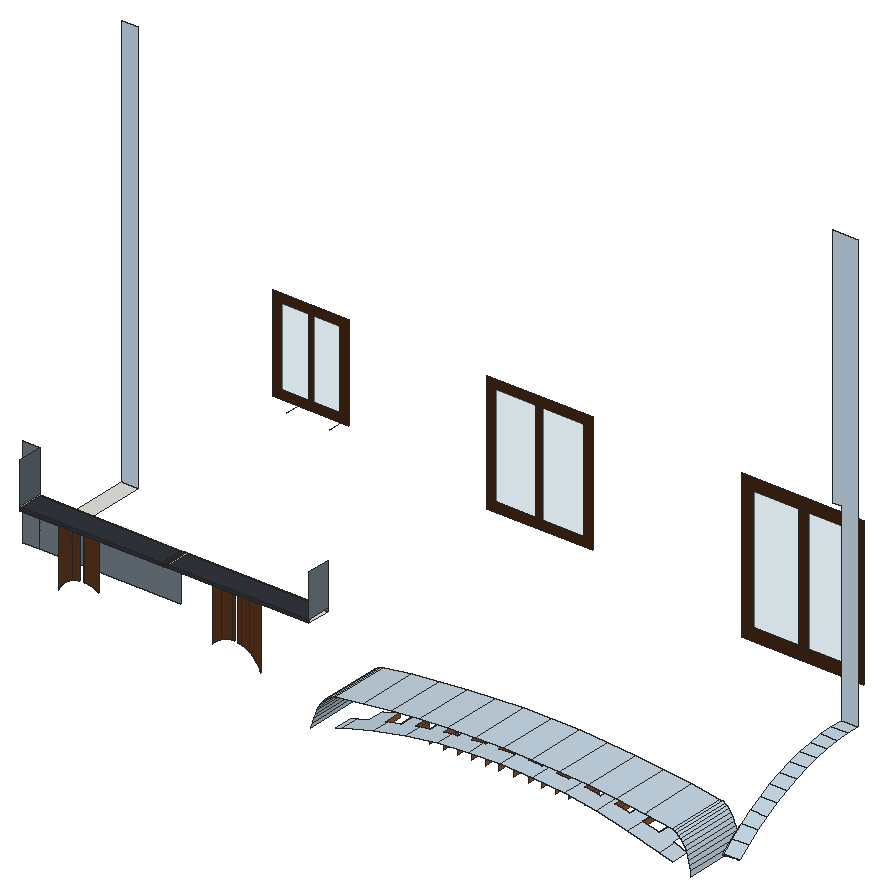
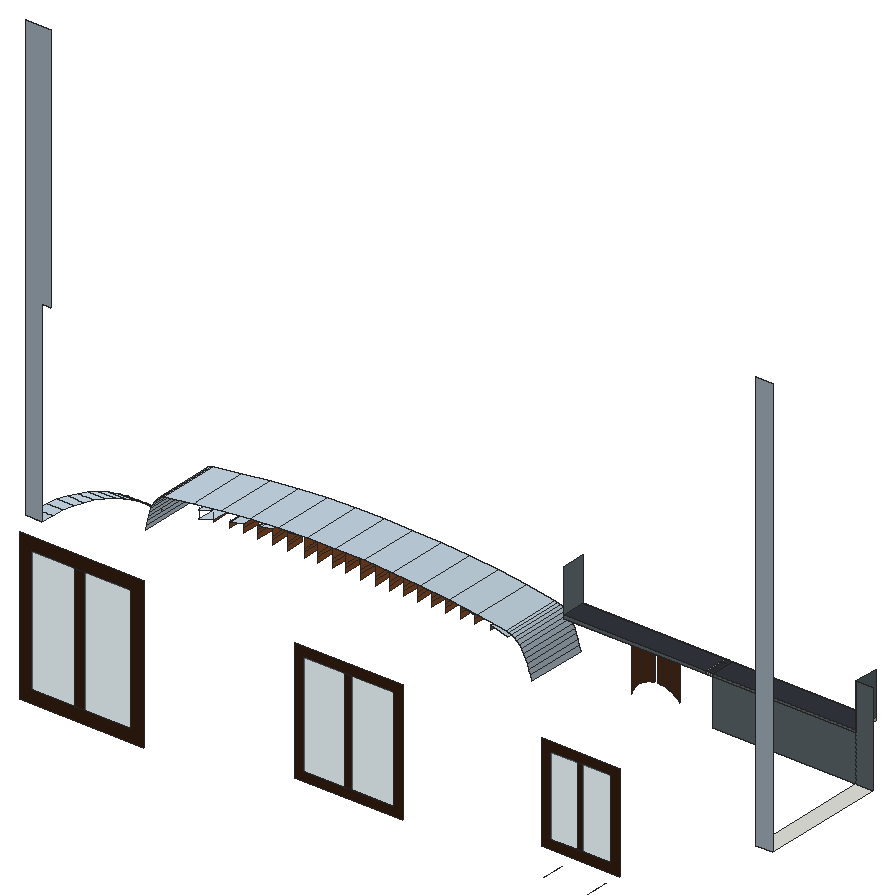
# SketchUp Ruby script. Lengths in inches.
U = 1.inch
M = Sketchup.active_model
def pt(a) = Geom::Point3d.new(a.map { |v| v * U })
def face(e, loops, mat)
  f = e.add_face(loops[0].map { |a| pt(a) })
  loops[1..].each { |l| e.add_face(l.map { |a| pt(a) }).erase! }
  f.material = f.back_material = mat if mat
  f
end
# faces: each face lists its corners as indices into pts; further lists are holes
def faces(e, pts, list, mat = nil) = list.each { |f| face(e, (f[0].is_a?(Array) ? f : [f]).map { |l| l.map { |i| pts[i] } }, mat) }
# xy, xz, yz: faces in a plane at the given z, y or x. An outline is a flat list of corners, or four numbers for a rectangle; further outlines are holes
def ring(l) = l.size == 4 ? [[l[0], l[1]], [l[2], l[1]], [l[2], l[3]], [l[0], l[3]]] : l.each_slice(2).to_a
def flat(e, list, mat, &to3) = list.each { |f| face(e, (f[0].is_a?(Array) ? f : [f]).map { |l| ring(l).map { |u, v| to3.(u, v) } }, mat) }
def xy(e, z, list, mat = nil) = flat(e, list, mat) { |x, y| [x, y, z] }
def xz(e, y, list, mat = nil) = flat(e, list, mat) { |x, z| [x, y, z] }
def yz(e, x, list, mat = nil) = flat(e, list, mat) { |y, z| [x, y, z] }
def lines(e, pts, list) = list.each { |a, b| e.add_line(pt(pts[a]), pt(pts[b])) }
# prism: a flat outline (further loops are holes) pulled along v
def prism(e, loops, v, mat = nil)
  f = face(e, loops, mat); d = Geom::Vector3d.new(v.map { |x| x * U })
  f.pushpull(f.normal.samedirection?(d) ? d.length : -d.length)
end
def box(e, o, s, mat = nil) = prism(e, [[o, [o[0] + s[0], o[1], o[2]], [o[0] + s[0], o[1] + s[1], o[2]], [o[0], o[1] + s[1], o[2]]]], [0, 0, s[2]], mat)
def at(x, y, z, deg = 0) = Geom::Transformation.translation(pt([x, y, z])) * Geom::Transformation.rotation(ORIGIN, Z_AXIS, deg.degrees)
def axes(o, x, y, z) = Geom::Transformation.new([*x, 0, *y, 0, *z, 0, *pt(o).to_a, 1])
def part(name) = M.definitions.add(name)
# library, detail: a bought-in or finely detailed component or shape, given as its bounding box
def library(name, o, s) = part(name).tap { |d| box(d.entities, o, s) }
def detail(e, o, s) = box(e.add_group.entities, o, s)
def put(e, d, t, mat = nil) = e.add_instance(d, t).tap { |i| i.material = mat if mat }
def group(e, t, mat = nil) = e.add_group.tap { |g| g.transformation = t; g.material = mat if mat }.entities
root = M.entities
M.materials.add("[Formica Laminate Dark]").color = [50, 53, 60]
M.materials.add("[Formica Speckled Grey]").color = [110, 123, 130]
M.materials.add("[Formica Speckled Grey]1").color = [94, 105, 111]
M.materials.add("[Terrazzo Light Blue]").color = [196, 214, 227]
M.materials.add("[Translucent Glass Safety]").color = [204, 235, 244]
M.materials["[Translucent Glass Safety]"].alpha = 0.5
M.materials.add("[Wood Cherry Original]").color = [152, 86, 42]
M.materials.add("[Wood Veneer 01]1").color = [86, 50, 26]
M.materials.add("[Wood Veneer 01]2").color = [63, 37, 19]
xy(root,128.61,[[0,134.14,19.68,283.27]])
xy(root,183.04,[[19.68,105.19,190.08,134.14],[190.08,105.19,198.05,134.14],[198.05,105.19,367.43,134.14]])
xy(root,186.5625,[[19.68,105.19,190.08,134.14],[190.08,105.19,193.18,134.14],[193.18,105.19,194.95,134.14],[194.95,105.19,198.05,134.14],[198.05,105.19,367.43,134.14]],"[Formica Laminate Dark]")
xz(root,105.19,[[868.09,108.42,887.77,109.72,868.09,109.72]])
xz(root,105.19,[[19.68,183.04,190.08,186.5625],[190.08,183.04,193.18,186.5625],[193.18,183.04,194.95,186.5625],[194.95,183.04,198.05,186.5625],[198.05,183.04,367.43,186.5625]],"[Formica Laminate Dark]")
xz(root,105.19,[[310.25,109.72,310.25,183.04,296.83,183.04,296.83,127.07,298.1,126.25,300.86,124.02,303.36,121.51,305.59,118.76,307.53,115.78,309.13,112.625],[65.75,113.31,65.96,113.76,66.33,114.49,66.71,115.2,67.11,115.91,67.53,116.61,67.97,117.3,68.42,117.97,68.88,118.64,69.37,119.29,69.87,119.93,70.38,120.5625,70.91,121.18,71.45,121.79,72.01,122.38,72.58,122.96,73.17,123.52,73.76,124.07,74.375,124.6,75,125.125,75.64,125.63,76.29,126.12,76.95,126.59,77.62,127.05,78.3,127.49,78.99,127.92,79.7,128.33,80.41,128.72,81.13,129.1,81.86,129.45,81.93,129.49,81.93,183.04,65.75,183.04],[252.33,120.67,253.01,121.51,255.52,124.02,258.28,126.25,261.25,128.18,263.46,129.31,263.46,183.04,252.33,183.04],[296.83,127.07,296.83,183.04,285.71,183.04,285.71,131.85,288.66,131.0625,291.97,129.79,295.125,128.18],[114.31,127.58,114.31,183.04,98.12,183.04,98.12,132.68,98.15,132.67,99.03,132.62,99.92,132.53,100.8,132.43,101.68,132.3,102.55,132.15,103.42,131.98,104.28,131.78,105.14,131.57,106,131.33,106.84,131.0625,107.68,130.78,108.52,130.47,109.34,130.14,110.15,129.79,110.96,129.42,111.75,129.03,112.54,128.62,113.3125,128.18,114.08,127.73],
  [263.46,129.31,264.41,129.79,267.72,131.0625,271.15,131.98,274.58,132.52,274.58,183.04,263.46,183.04],[81.93,129.49,82.6,129.79,83.34,130.11,84.1,130.42,84.86,130.7,85.63,130.97,86.4,131.22,87.18,131.45,87.97,131.66,88.76,131.85,89.55,132.03,90.35,132.18,91.15,132.31,91.99,132.14,91.99,183.04,81.93,183.04],[285.71,131.85,285.71,183.04,282.74,183.04,282.74,132.375,285.23,131.98],[274.58,132.52,274.65,132.53,278.1875,132.72,278.36,132.71,278.36,183.04,274.58,183.04],[98.12,132.68,98.12,183.04,96.375,183.04,96.375,132.72,97.26,132.71]],"[Wood Veneer 01]1")
xz(root,134.14,[[190.08,183.04,193.18,186.5625],[193.18,183.04,194.95,186.5625],[194.95,183.04,198.05,186.5625]])
xz(root,134.14,[[0,128.61,19.68,238.16],[19.68,128.61,190.08,183.04],[19.68,183.04,190.08,186.5625],[198.05,183.04,367.43,186.5625]],"[Formica Speckled Grey]")
xz(root,283.27,[[0,128.61,19.68,627.66],[868.09,175.78,887.77,175.78,887.77,702.66,857.52,702.66,857.52,407.22,868.09,407.22]],"[Terrazzo Light Blue]")
xz(root,454.3,[[625.86,115.33,680.16,263.36],[692.53,115.33,743.14,263.36],[313.91,142.1875,362.85,264.26],[371.15,142.1875,420.11,264.26],[55.54,172.47,88.73,266.53],
  [94.98,172.47,126.6,266.53]],"[Translucent Glass Safety]")
xz(root,454.3,[[[611.1,100.57,757.91,278.13],[625.86,115.33,743.14,263.36]],[680.16,115.33,692.53,263.36],[[303.04,131.32,430.98,275.13],[313.91,142.1875,420.11,264.26]],[362.85,142.1875,371.15,264.26],[[45.16,162.09,136.97,276.9],[55.54,172.47,126.6,266.53]],
  [88.73,172.47,94.98,266.53]],"[Wood Veneer 01]2")
yz(root,19.68,[[105.19,183.04,134.14,186.5625]])
yz(root,19.68,[[105.19,186.5625,134.14,238.16]],"[Formica Speckled Grey]1")
yz(root,190.08,[[105.19,183.04,134.14,186.5625]])
yz(root,198.05,[[105.19,183.04,134.14,186.5625]])
yz(root,367.43,[[105.19,186.5625,134.14,238.16]],"[Formica Speckled Grey]")
yz(root,477.51,[[84.44,119.05,105.19,124.6]],"[Wood Cherry Original]")
yz(root,495.83,[[84.44,119.05,105.19,124.6],[84.44,124.6,105.19,128.67]],"[Wood Cherry Original]")
yz(root,513.14,[[84.44,132.11,105.19,132.3]])
yz(root,513.14,[[84.44,119.05,105.19,124.6],[84.44,124.6,105.19,128.67],[84.44,128.67,105.19,132.11]],"[Wood Cherry Original]")
yz(root,530.58,[[84.44,119.05,105.19,124.6],[84.44,124.6,105.19,128.67],[84.44,128.67,105.19,135.3]],"[Wood Cherry Original]")
yz(root,547.58,[[84.44,119.05,105.19,124.6],[84.44,124.6,105.19,128.67],[84.44,128.67,105.19,137.84]],"[Wood Cherry Original]")
yz(root,564.14,[[84.44,119.05,105.19,124.6],[84.44,124.6,105.19,128.67],[84.44,128.67,105.19,139.94]],"[Wood Cherry Original]")
yz(root,580.83,[[84.44,119.05,105.19,124.6],[84.44,124.6,105.19,128.67],[84.44,128.67,105.19,141.4375]],"[Wood Cherry Original]")
yz(root,597.64,[[84.44,119.05,105.19,124.6],[84.44,124.6,105.19,128.67],[84.44,128.67,105.19,142.86]],"[Wood Cherry Original]")
yz(root,613.45,[[84.44,119.05,105.19,124.6],[84.44,124.6,105.19,128.67],[84.44,128.67,105.19,143.33]],"[Wood Cherry Original]")
yz(root,631.83,[[84.44,119.05,105.19,124.6],[84.44,124.6,105.19,128.67],[84.44,128.67,105.19,143.88]],"[Wood Cherry Original]")
yz(root,650.26,[[84.44,119.05,105.19,124.6],[84.44,124.6,105.19,128.67],[84.44,128.67,105.19,143.5]],"[Wood Cherry Original]")
yz(root,665.7,[[84.44,119.05,105.19,124.6],[84.44,124.6,105.19,128.67],[84.44,128.67,105.19,143.04]],"[Wood Cherry Original]")
yz(root,683.14,[[84.44,119.05,105.19,124.6],[84.44,124.6,105.19,128.67],[84.44,128.67,105.19,141.91]],"[Wood Cherry Original]")
yz(root,698.33,[[84.44,119.05,105.19,124.6],[84.44,124.6,105.19,128.67],[84.44,128.67,105.19,140.55]],"[Wood Cherry Original]")
yz(root,718.2,[[84.44,119.05,105.19,124.6],[84.44,124.6,105.19,128.67],[84.44,128.67,105.19,138.35]],"[Wood Cherry Original]")
yz(root,736.39,[[84.44,119.05,105.19,124.6],[84.44,124.6,105.19,128.67],[84.44,128.67,105.19,135.63]],"[Wood Cherry Original]")
yz(root,754.39,[[84.44,119.05,105.19,124.6],[84.44,124.6,105.19,128.67],[84.44,128.67,105.19,132.65]],"[Wood Cherry Original]")
yz(root,771.39,[[84.44,119.05,105.19,124.6],[84.44,124.6,105.19,128.67],[84.44,128.67,105.19,129.09]],"[Wood Cherry Original]")
yz(root,787.33,[[84.44,119.05,105.19,124.6],[84.44,124.6,105.19,125.74]],"[Wood Cherry Original]")
yz(root,806.7,[[84.44,119.05,105.19,120.53]],"[Wood Cherry Original]")
yz(root,868.09,[[105.19,108.42,105.19,109.72,118.73,120.31,130.3,128.41,118.54,119.63,107.97,110.74]])
p = [[405.48,134.14,102.81],[405.48,61.94,102.81],[406.89,61.94,108.68],[406.89,134.14,108.68],[863.19,134.14,108.38],[863.19,61.94,108.38],
  [863.71,61.94,102.81],[863.71,134.14,102.81],[862.36,134.14,113.8],[862.36,61.94,113.8],[408.5625,61.94,114.26],[408.5625,134.14,114.26],
  [887.77,105.19,109.72],[887.77,118.73,120.31],[868.09,118.73,120.31],[868.09,105.19,109.72],[825.83,61.94,115.36],[825.83,84.44,115.36],
  [841.21,84.44,110.27],[841.21,61.94,110.27],[435.4375,61.94,112.74],[435.4375,84.44,112.74],[443.36,84.44,115.36],[443.36,61.94,115.36],
  [861.24,134.14,118.99],[861.24,61.94,118.99],[410.48,61.94,119.51],[410.48,134.14,119.51],[457.01,84.44,119.05],[457.01,105.19,119.05],
  [477.51,105.19,124.6],[477.51,84.44,124.6],[481.41,84.44,125.65],[481.41,61.94,125.65],[787.78,61.94,125.65],[787.78,84.44,125.65],
  [806.7,84.44,120.53],[806.7,105.19,120.53],[823.96,105.19,115.87],[823.96,84.44,115.87],[859.83,134.14,123.88],[859.83,61.94,123.88],
  [412.62,61.94,124.4],[412.62,134.14,124.4],[887.77,132.61,130.03],[868.09,132.61,130.03],[868.09,130.3,128.41],[858.16,134.14,128.43],
  [858.16,61.94,128.43],[414.96,61.94,128.87],[414.96,134.14,128.87],[495.83,84.44,128.67],[495.83,105.19,128.67],[513.14,105.19,132.3],
  [513.14,84.44,132.3],[519.59,84.44,133.66],[519.59,61.94,133.66],[749.6,105.19,133.66],[754.39,105.19,132.65],[754.39,84.44,132.65],
  [771.39,84.44,129.09],[771.39,105.19,129.09],[787.33,105.19,125.74],[787.33,84.44,125.74],[749.6,61.94,133.66],[856.24,134.14,132.55],
  [856.24,61.94,132.55],[417.5,61.94,132.89],[417.5,134.14,132.89],[887.77,146.79,138.86],[868.09,146.79,138.86],[854.11,134.14,136.22],
  [854.11,61.94,136.22],[420.2,61.94,136.44],[420.2,134.14,136.44],[530.58,84.44,135.3],[530.58,105.19,135.3],[547.58,105.19,137.84],
  [547.58,84.44,137.84],[557.87,84.44,139.38],[557.87,61.94,139.38],[711.32,105.19,139.38],[718.2,105.19,138.35],[718.2,84.44,138.35],
  [736.39,84.44,135.63],[736.39,105.19,135.63],[711.32,61.94,139.38],[851.78,134.14,139.36],[851.78,61.94,139.36],[423.05,61.94,139.48],
  [423.05,134.14,139.48],[887.77,161.26,146.78],[868.09,161.26,146.78],[564.14,84.44,139.94],[564.14,105.19,139.94],[580.83,105.19,141.4375],
  [580.83,84.44,141.4375],[596.21,84.44,142.82],[596.21,61.94,142.82],[672.97,105.19,142.82],[683.14,105.19,141.91],[683.14,84.44,141.91],
  [698.33,84.44,140.55],[698.33,105.19,140.55],[672.97,61.94,142.82],[849.3,134.14,141.96],[849.3,61.94,141.96],[426.02,61.94,141.98],
  [426.02,134.14,141.98],[429.09,61.94,143.93],[429.09,134.14,143.93],[846.6875,134.14,143.96],[846.6875,61.94,143.96],[597.64,84.44,142.86],
  [597.64,105.19,142.86],[613.45,105.19,143.33],[613.45,84.44,143.33],[631.83,84.44,143.88],[631.83,105.19,143.88],[634.59,105.19,143.96],
  [634.59,61.94,143.96],[650.26,105.19,143.5],[650.26,84.44,143.5],[665.7,84.44,143.04],[665.7,105.19,143.04],[432.24,61.94,145.32],
  [432.24,134.14,145.32],[843.98,134.14,145.36],[843.98,61.94,145.36],[435.4375,61.94,146.12],[435.4375,134.14,146.12],[841.21,134.14,146.12],
  [841.21,61.94,146.12],[469.2,61.94,151.02],[469.2,134.14,151.02],[807.45,134.14,151.02],[807.45,61.94,151.02],[887.77,175.97,153.77],
  [868.09,175.97,153.77],[502.99,61.94,155.03],[502.99,134.14,155.03],[773.66,134.14,155.03],[773.66,61.94,155.03],[887.77,190.91,159.82],
  [868.09,190.91,159.82],[536.8,61.94,158.15],[536.8,134.14,158.15],[739.84,134.14,158.15],[739.84,61.94,158.15],[570.63,61.94,160.38],
  [570.63,134.14,160.38],[706.01,134.14,160.38],[706.01,61.94,160.38],[887.77,206.02,164.92],[868.09,206.02,164.92],[604.47,61.94,161.72],
  [604.47,134.14,161.72],[672.17,134.14,161.72],[672.17,61.94,161.72],[638.32,61.94,162.17],[638.32,134.14,162.17],[887.77,221.29,169.05],
  [868.09,221.29,169.05],[887.77,236.6875,172.21],[868.09,236.6875,172.21],[887.77,252.17,174.38],[868.09,252.17,174.38],[887.77,267.71,175.57],
  [868.09,267.71,175.57],[887.77,283.27,175.78],[868.09,283.27,175.78],[112.95,454.3,149.35],[112.95,482.57,149.35],[61.14,454.3,149.35],
  [61.14,482.57,149.35],[787.33,105.19,128.67],[806.7,105.19,125.74],[806.7,105.19,128.67],[806.7,105.19,124.6],[823.96,105.19,125.74],
  [823.96,105.19,128.67],[823.96,105.19,124.6],[823.96,105.19,119.05],[823.96,105.19,120.53]]
faces(root,p,[[0,1,2,3],[4,5,6,7],[8,9,5,4],[3,2,10,11],[12,13,14,15],[16,17,18,19],[20,21,22,23],[24,25,9,8],
  [11,10,26,27],[23,22,28,29,30,31,32,33],[34,35,36,37,38,39,17,16],[40,41,25,24],[27,26,42,43],[13,44,45,46,14],[47,48,41,40],[43,42,49,50],
  [33,32,51,52,53,54,55,56],[57,58,59,60,61,62,63,35,34,64],[65,66,48,47],[50,49,67,68],[44,69,70,45],[71,72,66,65],[68,67,73,74],[56,55,75,76,77,78,79,80],
  [81,82,83,84,85,57,64,86],[87,88,72,71],[74,73,89,90],[69,91,92,70],[80,79,93,94,95,96,97,98],[99,100,101,102,103,81,86,104],[105,106,88,87],[90,89,107,108],
  [108,107,109,110],[111,112,106,105],[98,97,113,114,115,116,117,118,119,120],[119,121,122,123,124,99,104,120],[110,109,125,126],[127,128,112,111],[126,125,129,130],[131,132,128,127],
  [130,129,133,134],[135,136,132,131],[91,137,138,92],[134,133,139,140],[141,142,136,135],[137,143,144,138],[140,139,145,146],[147,148,142,141],
  [146,145,149,150],[151,152,148,147],[143,153,154,144],[150,149,155,156],[157,158,152,151],[156,155,159,160],[160,159,158,157],[153,161,162,154],
  [161,163,164,162],[163,165,166,164],[165,167,168,166],[167,169,170,168]],"[Terrazzo Light Blue]")
lines(root,p,[[171,172],[173,174],[62,175],[176,177],[178,176],[37,178],[179,180],[181,179],[182,38],[182,183],[183,181]])
